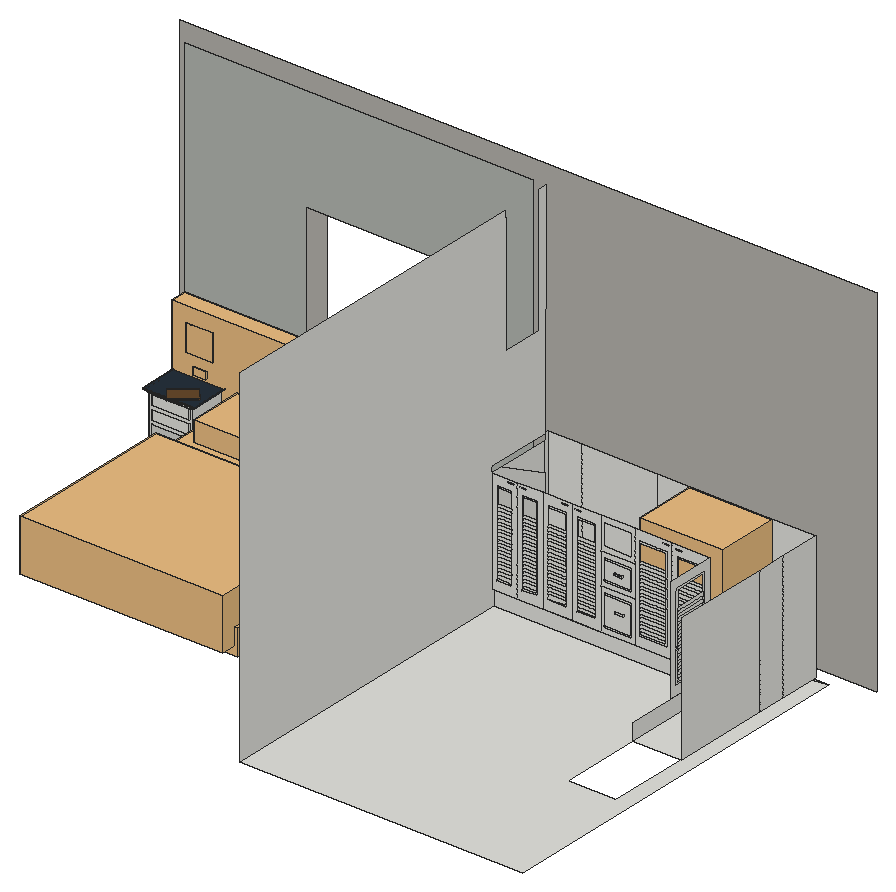
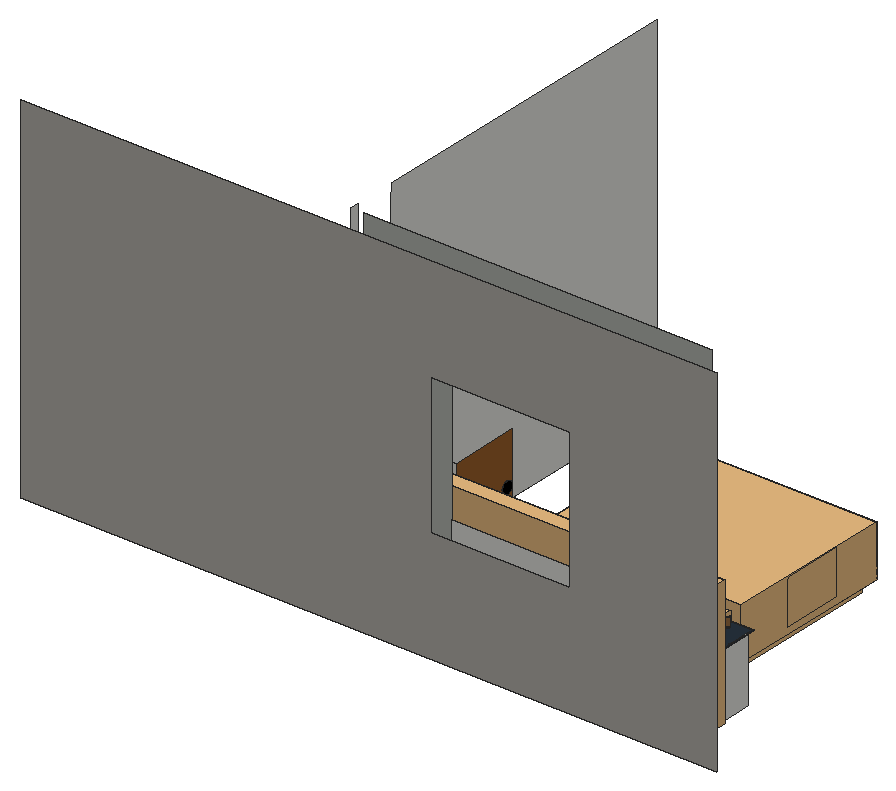
# SketchUp Ruby script. Lengths in inches.
U = 1.inch
M = Sketchup.active_model
def pt(a) = Geom::Point3d.new(a.map { |v| v * U })
def face(e, loops, mat)
  f = e.add_face(loops[0].map { |a| pt(a) })
  loops[1..].each { |l| e.add_face(l.map { |a| pt(a) }).erase! }
  f.material = f.back_material = mat if mat
  f
end
# faces: each face lists its corners as indices into pts; further lists are holes
def faces(e, pts, list, mat = nil) = list.each { |f| face(e, (f[0].is_a?(Array) ? f : [f]).map { |l| l.map { |i| pts[i] } }, mat) }
# xy, xz, yz: faces in a plane at the given z, y or x. An outline is a flat list of corners, or four numbers for a rectangle; further outlines are holes
def ring(l) = l.size == 4 ? [[l[0], l[1]], [l[2], l[1]], [l[2], l[3]], [l[0], l[3]]] : l.each_slice(2).to_a
def flat(e, list, mat, &to3) = list.each { |f| face(e, (f[0].is_a?(Array) ? f : [f]).map { |l| ring(l).map { |u, v| to3.(u, v) } }, mat) }
def xy(e, z, list, mat = nil) = flat(e, list, mat) { |x, y| [x, y, z] }
def xz(e, y, list, mat = nil) = flat(e, list, mat) { |x, z| [x, y, z] }
def yz(e, x, list, mat = nil) = flat(e, list, mat) { |y, z| [x, y, z] }
def lines(e, pts, list) = list.each { |a, b| e.add_line(pt(pts[a]), pt(pts[b])) }
# prism: a flat outline (further loops are holes) pulled along v
def prism(e, loops, v, mat = nil)
  f = face(e, loops, mat); d = Geom::Vector3d.new(v.map { |x| x * U })
  f.pushpull(f.normal.samedirection?(d) ? d.length : -d.length)
end
def box(e, o, s, mat = nil) = prism(e, [[o, [o[0] + s[0], o[1], o[2]], [o[0] + s[0], o[1] + s[1], o[2]], [o[0], o[1] + s[1], o[2]]]], [0, 0, s[2]], mat)
def at(x, y, z, deg = 0) = Geom::Transformation.translation(pt([x, y, z])) * Geom::Transformation.rotation(ORIGIN, Z_AXIS, deg.degrees)
def axes(o, x, y, z) = Geom::Transformation.new([*x, 0, *y, 0, *z, 0, *pt(o).to_a, 1])
def part(name) = M.definitions.add(name)
# library, detail: a bought-in or finely detailed component or shape, given as its bounding box
def library(name, o, s) = part(name).tap { |d| box(d.entities, o, s) }
def detail(e, o, s) = box(e.add_group.entities, o, s)
def put(e, d, t, mat = nil) = e.add_instance(d, t).tap { |i| i.material = mat if mat }
def group(e, t, mat = nil) = e.add_group.tap { |g| g.transformation = t; g.material = mat if mat }.entities
root = M.entities
M.materials.add("15___Default_0_2").color = [173, 175, 171]
M.materials.add("Material__1").color = [125, 118, 110]
M.materials.add("PDM Brown VP_Books_03").color = [85, 37, 1]
M.materials.add("PDM Cover VP_Books_03").color = [103, 73, 44]
M.materials.add("PDM Pages VP_Books_03").color = [224, 224, 224]
M.materials.add("W143X910B75_NILAYA NEW MODERN 31846 ROLL B75").color = [180, 183, 177]
M.materials.add("[Color M09]").color = [0, 0, 0]
M.materials.add("[Marble Carrara Gold Floor Tile]").color = [225, 223, 217]
M.materials.add("[Tile Travertine 2 inch]").color = [181, 178, 172]
M.materials.add("[Wood Floor Dark]").color = [153, 94, 42]
M.materials.add("wire_1").color = [39, 49, 60]
c1 = library("Group\#23",[-408.7,46.15,517.94],[1547.31,468.28,362.21])
c2 = library("Group\#21",[-519.15,-1391.32,251.35],[1756.04,1892.7,383.55])
c3 = library("Group\#20",[-576.09,-1463.59,4.12],[1840.9,2045.19,319.09])
c4 = library("Group\#19",[-609.9,-1576.45,97.75],[1838.77,1457.89,642.22])
c5 = library("Group\#12",[-612.85,-1140.67,180.96],[1888,514.01,543.34])
c6 = library("Group\#15",[-455.57,-1315.72,309.1],[1631.9,1798.78,127.41])
c7 = part("BED-0235")
put(c7.entities,c1,at(0,0,0),"wire_1")
g1 = group(c7.entities,at(0,0,0),"wire_1")
p = [[710.91,736.79,563.57],[711.15,735.84,567.82],[713.76,733.43,565.7],[231.46,704.77,566.08],[225.3,708.01,564.82],[226.88,706.82,568.1875],
  [225.36,706.93,576.125]]
faces(g1,p,[[0,1,2],[3,4,5],[6,3,5]],"15___Default_0_2")
put(c7.entities,c2,at(0,0,0),"wire_1")
put(c7.entities,c3,at(0,0,0),"wire_1")
put(c7.entities,c4,at(0,0,0),"wire_1")
put(c7.entities,c5,at(0,0,0),"Material__1")
put(c7.entities,c6,at(0,0,0),"wire_1")
c8 = part("VP_Books_03_Cover")
xy(c8.entities,-0.33,[[0,-1.3,11.69,7.49]],"PDM Brown VP_Books_03")
xy(c8.entities,-0.25,[[0,-1.22,11.69,7.49]],"PDM Brown VP_Books_03")
xy(c8.entities,1.04,[[0,-1.22,11.69,7.49]],"PDM Brown VP_Books_03")
xy(c8.entities,1.12,[[0,-1.3,11.69,7.49]],"PDM Cover VP_Books_03")
xz(c8.entities,-1.3,[[0,-0.33,11.69,1.12]],"PDM Cover VP_Books_03")
xz(c8.entities,-1.22,[[0,-0.25,11.69,1.04]],"PDM Brown VP_Books_03")
xz(c8.entities,7.49,[[0,-0.33,11.69,-0.25],[0,1.04,11.69,1.12]],"PDM Brown VP_Books_03")
yz(c8.entities,0,[[-1.3,-0.33,-1.3,1.12,7.49,1.12,7.49,1.04,-1.22,1.04,-1.22,-0.25,7.49,-0.25,7.49,-0.33]],"PDM Cover VP_Books_03")
yz(c8.entities,11.69,[[-1.3,-0.33,7.49,-0.33,7.49,-0.25,-1.22,-0.25,-1.22,1.04,7.49,1.04,7.49,1.12,-1.3,1.12]],"PDM Cover VP_Books_03")
c9 = part("VP_Books_03_Pages")
box(c9.entities,[0,-1.3,-0.33],[11.46,8.59,1.29],"PDM Pages VP_Books_03")
c10 = part("VP_Books_03.skp")
put(c10.entities,c8,axes([0,1.57,0.39],[1.21,0,0],[0,1.21,0],[0,0,1.21]))
put(c10.entities,c9,axes([0.14,1.67,0.49],[1.21,0,0],[0,1.21,0],[0,0,1.21]))
c11 = part("Chevet CHENONCEAU, Maisons du monde. Réf: 115.709 Prix: 129")
xy(c11.entities,0,[[1.3125,0.79,2.43,12.99],[15.54,0.79,16.57,12.99]])
xy(c11.entities,2.03,[[4.39,0.79,13.68,12.99]])
xy(c11.entities,3.26,[[2.51,0.79,15.51,12.52]])
xy(c11.entities,12.82,[[2.51,0.79,15.51,12.52]])
xy(c11.entities,14.17,[[2.51,0.67,15.42,0.79]])
xy(c11.entities,17.37,[[2.51,0.67,15.42,0.79]])
xy(c11.entities,18.73,[[2.53,0.72,15.34,0.79]])
xy(c11.entities,21.96,[[2.53,0.72,15.34,0.79]])
xy(c11.entities,22.57,[[1.3125,0.39,16.57,0.79],[16.57,0.39,16.89,12.99]])
xy(c11.entities,23.26,[[0,0,0.79,12.99],[0.79,0,17.11,0.39],[17.11,0,17.72,12.99]])
xy(c11.entities,23.62,[[0,0,17.72,12.99]],"wire_1")
xz(c11.entities,0,[[0,23.26,17.72,23.62]],"wire_1")
xz(c11.entities,0.39,[[1.3125,22.57,16.89,22.57,17.11,23.11,0.79,23.09],[0.79,23.09,17.11,23.11,17.11,23.26,0.79,23.26]])
xz(c11.entities,0.67,[[2.51,14.17,15.42,17.37]])
xz(c11.entities,0.72,[[2.53,18.73,15.34,21.96]])
xz(c11.entities,0.79,[[[1.3125,0,2.43,0,2.44,0.26,2.48,0.52,2.56,0.77,2.67,1.01,2.81,1.23,2.98,1.43,3.17,1.61,3.39,1.76,3.62,1.875,3.87,1.96,4.125,2.01,4.39,2.03,13.68,2.03,13.9375,2.01,14.1875,1.96,14.43,1.875,14.66,1.75,14.87,1.6,15.06,1.43,15.22,1.22,15.35,1,15.45,0.76,15.51,0.51,15.54,0.26,15.54,0,16.57,0,16.57,22.57,1.3125,22.57],[2.51,3.26,15.51,12.82],[2.53,18.73,15.34,21.96],[2.51,14.17,15.42,17.37]]])
xz(c11.entities,12.52,[[2.51,3.26,15.51,12.82]])
xz(c11.entities,12.99,[[1.3125,0,1.3125,22.57,0.79,23.09,0.79,23.26,0,23.26,0,23.62,17.72,23.62,17.72,23.26,17.11,23.26,17.11,23.11,16.89,22.57,16.57,22.57,16.57,0,15.54,0,15.54,0.26,15.51,0.51,15.45,0.76,15.35,1,15.22,1.22,15.06,1.43,14.87,1.6,14.66,1.75,14.43,1.875,14.1875,1.96,13.9375,2.01,13.68,2.03,4.39,2.03,4.125,2.01,3.87,1.96,3.62,1.875,3.39,1.76,3.17,1.61,2.98,1.43,2.81,1.23,2.67,1.01,2.56,0.77,2.48,0.52,2.44,0.26,2.43,0]])
yz(c11.entities,0,[[0,23.26,12.99,23.62]],"wire_1")
yz(c11.entities,0.79,[[0.39,23.09,12.99,23.26]])
yz(c11.entities,1.3125,[[0.79,0,12.99,22.57]])
yz(c11.entities,2.51,[[0.79,3.26,12.52,12.82],[0.67,14.17,0.79,17.37]])
yz(c11.entities,2.53,[[0.72,18.73,0.79,21.96]])
yz(c11.entities,15.34,[[0.72,18.73,0.79,21.96]])
yz(c11.entities,15.42,[[0.67,14.17,0.79,17.37]])
yz(c11.entities,15.51,[[0.79,3.26,12.52,12.82]])
yz(c11.entities,15.54,[[0.79,0,12.99,0.26]])
yz(c11.entities,16.57,[[0.79,0,12.99,22.57]])
yz(c11.entities,17.11,[[0.39,23.11,12.99,23.26]])
yz(c11.entities,17.72,[[0,23.26,12.99,23.62]],"wire_1")
p = [[2.43,12.99,0],[2.44,12.99,0.26],[2.44,0.79,0.26],[2.43,0.79,0],[2.48,12.99,0.52],[2.48,0.79,0.52],
  [15.51,12.99,0.51],[15.54,12.99,0.26],[15.54,0.79,0.26],[15.51,0.79,0.51],[2.56,12.99,0.77],[2.56,0.79,0.77],
  [15.45,12.99,0.76],[15.45,0.79,0.76],[2.67,12.99,1.01],[2.67,0.79,1.01],[15.35,12.99,1],[15.35,0.79,1],
  [2.81,12.99,1.23],[2.81,0.79,1.23],[15.22,12.99,1.22],[15.22,0.79,1.22],[2.98,12.99,1.43],[2.98,0.79,1.43],
  [15.06,12.99,1.43],[15.06,0.79,1.43],[3.17,12.99,1.61],[3.17,0.79,1.61],[14.87,12.99,1.6],[14.87,0.79,1.6],
  [3.39,12.99,1.76],[3.39,0.79,1.76],[14.66,12.99,1.75],[14.66,0.79,1.75],[3.62,12.99,1.875],[3.62,0.79,1.875],
  [14.43,12.99,1.875],[14.43,0.79,1.875],[3.87,12.99,1.96],[3.87,0.79,1.96],[14.1875,12.99,1.96],[14.1875,0.79,1.96],
  [4.125,12.99,2.01],[4.125,0.79,2.01],[4.39,12.99,2.03],[4.39,0.79,2.03],[13.68,12.99,2.03],[13.9375,12.99,2.01],
  [13.9375,0.79,2.01],[13.68,0.79,2.03],[1.3125,0.79,22.57],[1.3125,0.39,22.57],[0.79,0.39,23.09],[0.79,12.99,23.09],
  [1.3125,12.99,22.57],[17.11,12.99,23.11],[17.11,0.39,23.11],[16.89,0.39,22.57],[16.89,12.99,22.57]]
faces(c11.entities,p,[[0,1,2,3],[1,4,5,2],[6,7,8,9],[4,10,11,5],[12,6,9,13],[10,14,15,11],[16,12,13,17],[14,18,19,15],
  [20,16,17,21],[18,22,23,19],[24,20,21,25],[22,26,27,23],[28,24,25,29],[26,30,31,27],[32,28,29,33],[30,34,35,31],
  [36,32,33,37],[34,38,39,35],[40,36,37,41],[38,42,43,39],[42,44,45,43],[46,47,48,49],[47,40,41,48],[50,51,52,53,54],
  [55,56,57,58]])
c12 = library("Alarm_clock_retro.skp",[-0.85,-1.11,-0.01],[5.38,3.78,6.48])
c13 = part("Sink_Counter_Double")
detail(c13.entities,[0,0,-12],[39,21,12.25])
c14 = library("ELK",[8.53,-0.73,3.43],[4.44,1.03,2.5])
c15 = library("Bega_2263.skp",[0,0,-4.33],[9.1,9.1,4.54])
xy(root,38.43,[[[133.5,303,231,303,231,435,225.68,434.1875,225.68,431.8,133.5,431.8],[208.97,349.92,225.68,378.03]],[133.5,431.8,145.02,434.1875],[145.02,431.8,170.95,434.1875],[170.95,431.8,182.47,434.1875],[182.47,431.8,208.39,434.1875],
  [208.39,431.8,225.68,434.1875],[133.5,434.1875,145.02,434.1875,145.02,434.28],[133.5,434.1875,145.02,434.28,145.02,435.8125,133.5,435.8125],[145.02,434.1875,170.95,434.1875,170.95,434.5,145.02,434.28],[170.95,434.1875,182.47,434.1875,182.47,434.59,170.95,434.5],
  [182.47,434.1875,208.39,434.1875,208.39,434.8125,182.47,434.59],[208.39,434.1875,225.68,434.1875,225.68,434.96,208.39,434.8125],[225.68,434.1875,231,435,225.68,434.96],[145.02,434.28,170.95,434.5,170.95,435.8125,145.02,435.8125],[170.95,434.5,182.47,434.59,182.47,435.8125,170.95,435.8125],
  [182.47,434.59,208.39,434.8125,208.39,435.8125,182.47,435.8125],[208.39,434.8125,225.68,434.96,225.68,435.8125,208.39,435.8125]])
xy(root,43.89,[[208.39,394.875,208.97,411.72],[133.5,411.72,145.02,412.52],[145.02,411.72,157.98,412.52],[157.98,411.72,170.95,412.52],[170.95,411.72,182.47,412.52],
  [182.47,411.72,195.43,412.52],[195.43,411.72,208.97,412.52]])
xy(root,51.36,[[175.87,411.4,178.72,411.72]])
xy(root,51.91,[[175.87,411.4,178.72,411.72]])
xy(root,63.14,[[175.59,411.4,178.44,411.72]])
xy(root,63.68,[[175.59,411.4,178.44,411.72]])
xz(root,409.98,[[117,38.43,129,74.43]],"[Marble Carrara Gold Floor Tile]")
xz(root,411.4,[[175.87,51.36,178.72,51.91],[175.59,63.14,178.44,63.68]])
xz(root,411.72,[[[133.5,43.89,142.14,79.89],[135.23,47.16,140.41,76.61],[138.5625,78.57,141.42,79.12]],[[142.14,43.89,150.78,79.89],[143.87,47.16,149.05,76.61],[142.6,78.52,145.45,79.07]],[[150.78,43.89,160.86,79.89],[152.51,47.16,159.14,76.61],[157.16,78.54,160.01,79.08]],[[160.86,43.89,170.95,79.89],[162.59,47.16,169.22,76.61],[161.46,78.41,164.3125,78.96]],[[170.95,43.89,182.47,58.07],[171.8125,45.52,181.6,56.43]],
  [[182.47,43.89,195.43,79.89],[184.2,47.16,193.7,76.61],[191.81,78.52,194.66,79.06]],[[195.43,43.89,208.39,79.89],[197.16,47.16,206.67,76.61],[196.33,78.19,199.18,78.74]],[[171.8125,45.52,181.6,56.43],[172.1,46.07,181.32,55.89]],[[172.1,46.07,181.32,55.89],[175.87,51.36,178.72,51.91]],[[135.23,47.16,140.41,76.61],[135.52,47.7,140.125,76.07]],
  [[143.87,47.16,149.05,76.61],[144.16,47.7,148.77,76.07]],[[152.51,47.16,159.14,76.61],[152.8,47.7,158.85,76.07]],[[162.59,47.16,169.22,76.61],[162.88,47.7,168.93,76.07]],[[184.2,47.16,193.7,76.61],[184.49,47.7,193.41,76.07]],[[197.16,47.16,206.67,76.61],[197.45,47.7,206.38,76.07]],
  [135.52,47.7,140.125,49.13],[144.16,47.7,148.77,48.79],[152.8,47.7,158.85,49.1],[162.88,47.7,168.93,48.79],[184.49,47.7,193.41,48.79],
  [197.45,47.7,206.38,48.79],[144.16,48.79,148.77,49.89],[162.88,48.79,168.93,49.89],[184.49,48.79,193.41,49.89],[197.45,48.79,206.38,49.89],
  [152.8,49.1,158.85,50.1875],[135.52,49.13,140.125,50.22],[144.16,49.89,148.77,50.98],[162.88,49.89,168.93,50.98],[184.49,49.89,193.41,50.98],
  [197.45,49.89,206.38,50.98],[152.8,50.1875,158.85,51.28],[135.52,50.22,140.125,51.3125],[144.16,50.98,148.77,52.07],[162.88,50.98,168.93,52.07],
  [184.49,50.98,193.41,52.07],[197.45,50.98,206.38,52.07],[152.8,51.28,158.85,52.37],[135.52,51.3125,140.125,52.4],[144.16,52.07,148.77,53.16],
  [162.88,52.07,168.93,53.16],[184.49,52.07,193.41,53.16],[197.45,52.07,206.38,53.16],[152.8,52.37,158.85,53.46],[135.52,52.4,140.125,53.49],
  [144.16,53.16,148.77,54.25],[162.88,53.16,168.93,54.25],[184.49,53.16,193.41,54.25],[197.45,53.16,206.38,54.25],[152.8,53.46,158.85,54.55],
  [135.52,53.49,140.125,54.58],[144.16,54.25,148.77,55.34],[162.88,54.25,168.93,55.34],[184.49,54.25,193.41,55.34],[197.45,54.25,206.38,55.34],
  [152.8,54.55,158.85,55.64],[135.52,54.58,140.125,55.68],[144.16,55.34,148.77,56.43],[162.88,55.34,168.93,56.43],[184.49,55.34,193.41,56.43],
  [197.45,55.34,206.38,56.43],[152.8,55.64,158.85,56.73],[135.52,55.68,140.125,56.77],[144.16,56.43,148.77,57.52],[162.88,56.43,168.93,57.52],
  [184.49,56.43,193.41,57.52],[197.45,56.43,206.38,57.52],[152.8,56.73,158.85,57.82],[135.52,56.77,140.125,57.86],[144.16,57.52,148.77,58.61],
  [162.88,57.52,168.93,58.61],[184.49,57.52,193.41,58.61],[197.45,57.52,206.38,58.61],[152.8,57.82,158.85,58.91],[135.52,57.86,140.125,58.95],
  [[170.95,58.07,182.47,68.98],[171.8125,59.7,181.6,67.34]],[144.16,58.61,148.77,59.7],[162.88,58.61,168.93,59.7],[184.49,58.61,193.41,59.7],[197.45,58.61,206.38,59.7],
  [152.8,58.91,158.85,60],[135.52,58.95,140.125,60.04],[144.16,59.7,148.77,60.79],[162.88,59.7,168.93,60.79],[[171.8125,59.7,181.6,67.34],[172.1,60.25,181.32,66.79]],
  [184.49,59.7,193.41,60.79],[197.45,59.7,206.38,60.79],[152.8,60,158.85,61.1],[135.52,60.04,140.125,61.13],[[172.1,60.25,181.32,66.79],[175.59,63.14,178.44,63.68]],
  [144.16,60.79,148.77,61.89],[162.88,60.79,168.93,61.89],[184.49,60.79,193.41,61.89],[197.45,60.79,206.38,61.89],[152.8,61.1,158.85,62.1875],
  [135.52,61.13,140.125,62.22],[144.16,61.89,148.77,62.98],[162.88,61.89,168.93,62.98],[184.49,61.89,193.41,62.98],[197.45,61.89,206.38,62.98],
  [152.8,62.1875,158.85,63.28],[135.52,62.22,140.125,63.3125],[144.16,62.98,148.77,64.07],[162.88,62.98,168.93,64.07],[184.49,62.98,193.41,64.07],
  [197.45,62.98,206.38,64.07],[152.8,63.28,158.85,64.37],[135.52,63.3125,140.125,64.4],[144.16,64.07,148.77,65.16],[162.88,64.07,168.93,65.16],
  [184.49,64.07,193.41,65.16],[197.45,64.07,206.38,65.16],[152.8,64.37,158.85,65.46],[135.52,64.4,140.125,65.49],[144.16,65.16,148.77,66.25],
  [162.88,65.16,168.93,66.25],[184.49,65.16,193.41,66.25],[197.45,65.16,206.38,66.25],[152.8,65.46,158.85,66.55],[135.52,65.49,140.125,66.58],
  [144.16,66.25,148.77,67.34],[162.88,66.25,168.93,67.34],[184.49,66.25,193.41,67.34],[197.45,66.25,206.38,67.34],[152.8,66.55,158.85,67.64],
  [135.52,66.58,140.125,67.68],[144.16,67.34,148.77,68.43],[162.88,67.34,168.93,68.43],[184.49,67.34,193.41,68.43],[197.45,67.34,206.38,68.43],
  [152.8,67.64,158.85,68.73],[135.52,67.68,140.125,68.77],[144.16,68.43,148.77,69.52],[162.88,68.43,168.93,69.52],[184.49,68.43,193.41,69.52],
  [197.45,68.43,206.38,69.52],[152.8,68.73,158.85,69.82],[135.52,68.77,140.125,69.86],[[170.95,68.98,182.47,79.89],[171.8125,70.61,181.6,78.25]],[144.16,69.52,148.77,70.61],
  [162.88,69.52,168.93,70.61],[184.49,69.52,193.41,70.61],[197.45,69.52,206.38,70.61],[152.8,69.82,158.85,70.91],[135.52,69.86,140.125,70.95]])
xz(root,412.52,[[133.5,38.43,208.97,43.89]])
xz(root,435,[[50.67,38.43,98.67,74.43]])
xz(root,435,[[9,38.43,50.67,38.43,50.67,122.43,98.67,122.43,98.67,38.43,129,38.43,129,158.43,9,158.43]],"W143X910B75_NILAYA NEW MODERN 31846 ROLL B75")
xz(root,435.8125,[[133.5,38.43,145.02,82.07],[145.02,38.43,170.95,82.07],[170.95,38.43,182.47,82.07],[182.47,38.43,208.39,82.07],[208.39,38.43,225.68,82.07]])
xz(root,444,[[[0,35.43,240,158.43],[50.67,74.43,98.67,122.43]]],"[Tile Travertine 2 inch]")
yz(root,116.5,[[388.58,55.67,388.06,55.74,387.58,55.95,387.17,56.26,386.85,56.68,386.65,57.16,386.59,57.68,386.66,58.2,386.86,58.68,387.18,59.09,387.59,59.41,388.07,59.61,388.59,59.67,389.11,59.61,389.59,59.4,390.01,59.09,390.32,58.67,390.52,58.1875,390.59,57.67,390.52,57.15,390.32,56.67,390,56.26,389.58,55.94,389.1,55.74]],"[Color M09]")
yz(root,117,[[[385.98,38.43,409.98,74.43],[388.58,55.67,389.1,55.74,389.58,55.94,390,56.26,390.32,56.67,390.52,57.15,390.59,57.67,390.52,58.1875,390.32,58.67,390.01,59.09,389.59,59.4,389.11,59.61,388.59,59.67,388.07,59.61,387.59,59.41,387.18,59.09,386.86,58.68,386.66,58.2,386.59,57.68,386.65,57.16,386.85,56.68,387.17,56.26,387.58,55.95,388.06,55.74]]],"[Wood Floor Dark]")
yz(root,133.5,[[303,38.43,412.52,38.43,412.52,43.89,411.72,43.89,411.72,79.89,411.55,79.98,411.41,80.12,411.28,80.29,411.19,80.5,411.14,80.73,411.12,80.98,411.14,81.22,411.19,81.45,411.28,81.66,411.41,81.84,411.55,81.97,411.72,82.07,434.1875,82.07,435,158.43,431.8,158.43,431.8,114.79,417.74,114.79,417.74,155.7,416.94,155.7,416.94,158.43,303,158.43],[412.52,38.43,434.1875,38.43,434.1875,69.93,415.76,79.89,411.72,79.89,411.72,43.89,412.52,43.89],[434.1875,38.43,435.8125,38.43,435.8125,82.07,435.01,82.07,435.01,79.89,434.1875,79.89],[434.1875,69.93,434.1875,79.89,415.76,79.89]])
yz(root,175.59,[[411.4,63.14,411.72,63.68]])
yz(root,175.87,[[411.4,51.36,411.72,51.91]])
yz(root,178.44,[[411.4,63.14,411.72,63.68]])
yz(root,178.72,[[411.4,51.36,411.72,51.91]])
yz(root,208.39,[[[394.875,43.89,411.72,79.89],[397.28,47.16,409.31,76.61]],[397.28,47.16,409.31,47.16,409.31,76.61,397.28,76.61,397.28,58.61,397.95,58.61,397.95,76.07,408.91,76.07,408.91,47.7,397.95,47.7,397.95,57.52,397.28,57.52],[397.95,47.7,408.91,48.79],[397.95,48.79,408.91,49.89],[397.95,49.89,408.91,50.98],
  [397.95,50.98,408.91,52.07],[397.95,52.07,408.91,53.16],[397.95,53.16,408.91,54.25],[397.95,54.25,408.91,55.34],[397.95,55.34,408.91,56.43],
  [397.95,56.43,408.91,57.52],[397.28,57.52,397.95,58.61],[397.95,57.52,408.91,58.61],[397.95,58.61,408.91,59.7],[397.95,59.7,408.91,60.79],
  [397.95,60.79,408.91,61.89],[397.95,61.89,408.91,62.98],[397.95,62.98,408.91,64.07],[397.95,64.07,408.91,65.16],[397.95,65.16,408.91,66.25],
  [397.95,66.25,408.91,67.34],[397.95,67.34,408.91,68.43],[397.95,68.43,408.91,69.52],[397.95,69.52,408.91,70.61]])
yz(root,208.97,[[378.03,38.43,412.52,43.89]])
yz(root,225.68,[[378.03,38.43,411.72,82.07],[411.72,38.43,421.76,82.07],[421.76,38.43,435.8125,82.07]])
p = [[117,388.58,55.67],[117,388.06,55.74],[116.5,388.06,55.74],[116.5,388.58,55.67],[117,389.1,55.74],[116.5,389.1,55.74],
  [117,389.58,55.94],[116.5,389.58,55.94],[117,390,56.26],[116.5,390,56.26],[117,390.32,56.67],[116.5,390.32,56.67],
  [117,390.52,57.15],[116.5,390.52,57.15],[117,390.59,57.67],[116.5,390.59,57.67],[117,390.52,58.1875],[116.5,390.52,58.1875],
  [117,390.32,58.67],[116.5,390.32,58.67],[117,390.01,59.09],[116.5,390.01,59.09],[117,389.59,59.4],[116.5,389.59,59.4],
  [117,389.11,59.61],[116.5,389.11,59.61],[117,388.07,59.61],[117,388.59,59.67],[116.5,388.59,59.67],[116.5,388.07,59.61],
  [94.12,351.58,38.81],[94.12,427.17,38.81],[17.74,427.17,39.99],[31.125,427.17,39.99],[94.12,427.17,39.99],[113.02,427.17,39.99]]
faces(root,p,[[0,1,2,3],[4,0,3,5],[6,4,5,7],[8,6,7,9],[10,8,9,11],[12,10,11,13],[14,12,13,15],[16,14,15,17],
  [18,16,17,19],[20,18,19,21],[22,20,21,23],[24,22,23,25],[26,27,28,29],[27,24,25,28]],"[Color M09]")
lines(root,p,[[30,31],[32,33],[33,34],[34,35]])
detail(root,[10.78,427.17,38.81],[103.42,5.51,44.48])
put(root,c7,axes([49.19,406.07,38.4],[0.03797,0,0],[0,0.0401,0],[0,0,0.02765]))
put(root,c10,axes([20.68,412.84,62.05],[0.46675,0.39584,0],[-0.34834,0.41074,0],[0,0,0.17]))
put(root,c11,at(11.16,414.27,38.43))
put(root,c11,at(95.42,414.27,38.43))
put(root,c12,at(101.76,420.08,62.05))
put(root,c13,axes([182.81,413.59,82.07],[0.73165,0,0],[0,1.02,0],[0,0,1.38545]))
put(root,c14,at(94.24,427.26,59.59))
put(root,c14,at(9.98,427.26,59.59))
put(root,c15,axes([100.09,427.17,69.03],[1,0,0],[0,0,1],[0,-1,0]))
put(root,c15,axes([15.84,427.17,69.03],[1,0,0],[0,0,1],[0,-1,0]))
